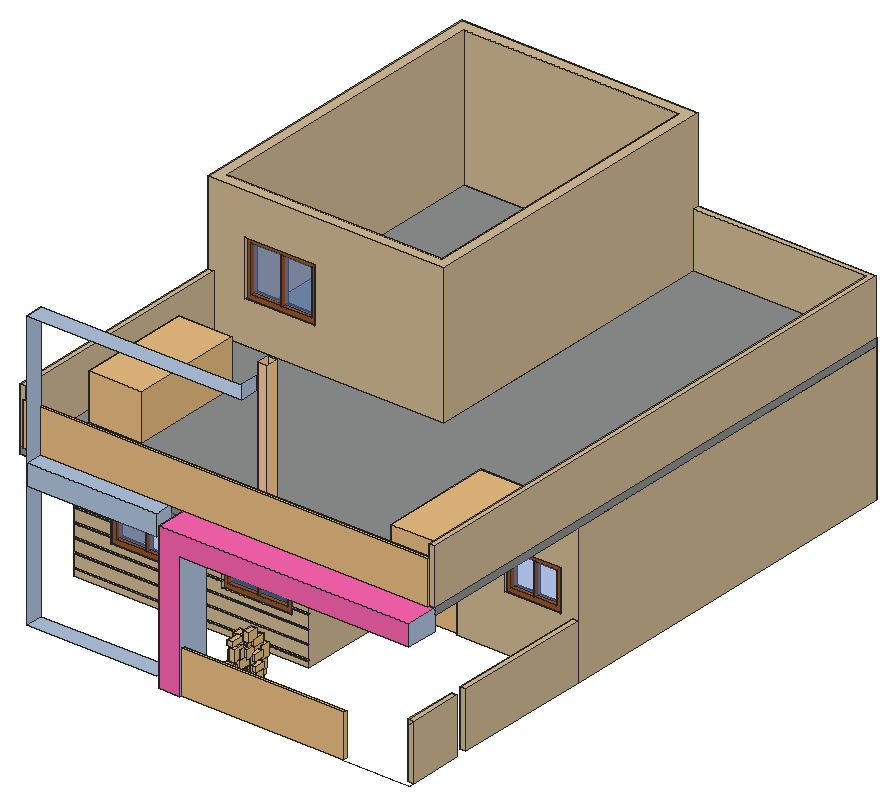
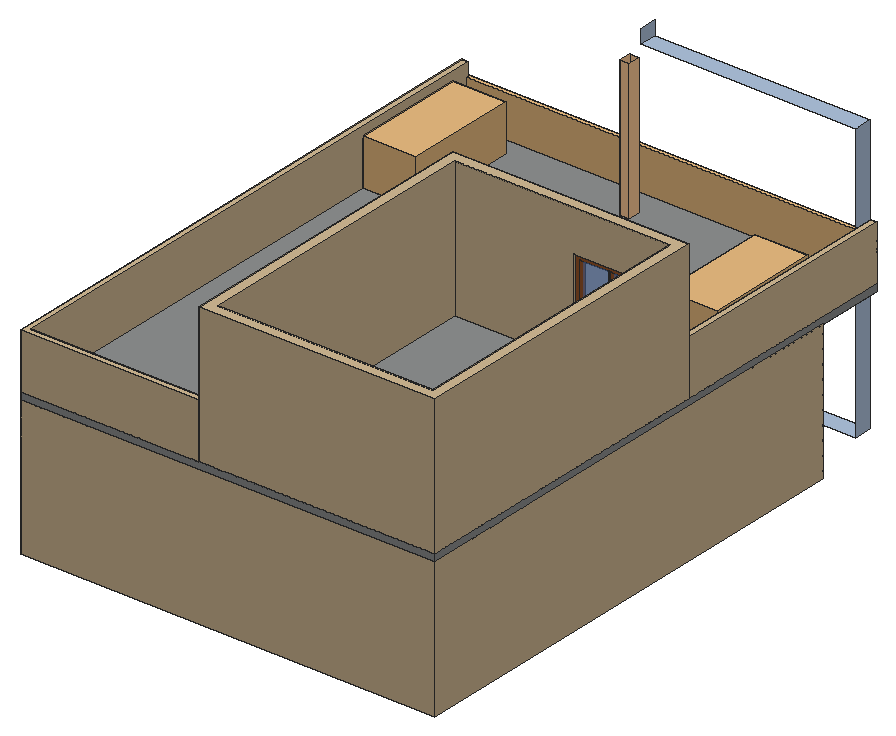
# SketchUp Ruby script. Lengths in inches.
U = 1.inch
M = Sketchup.active_model
def pt(a) = Geom::Point3d.new(a.map { |v| v * U })
def face(e, loops, mat)
  f = e.add_face(loops[0].map { |a| pt(a) })
  loops[1..].each { |l| e.add_face(l.map { |a| pt(a) }).erase! }
  f.material = f.back_material = mat if mat
  f
end
# faces: each face lists its corners as indices into pts; further lists are holes
def faces(e, pts, list, mat = nil) = list.each { |f| face(e, (f[0].is_a?(Array) ? f : [f]).map { |l| l.map { |i| pts[i] } }, mat) }
# xy, xz, yz: faces in a plane at the given z, y or x. An outline is a flat list of corners, or four numbers for a rectangle; further outlines are holes
def ring(l) = l.size == 4 ? [[l[0], l[1]], [l[2], l[1]], [l[2], l[3]], [l[0], l[3]]] : l.each_slice(2).to_a
def flat(e, list, mat, &to3) = list.each { |f| face(e, (f[0].is_a?(Array) ? f : [f]).map { |l| ring(l).map { |u, v| to3.(u, v) } }, mat) }
def xy(e, z, list, mat = nil) = flat(e, list, mat) { |x, y| [x, y, z] }
def xz(e, y, list, mat = nil) = flat(e, list, mat) { |x, z| [x, y, z] }
def yz(e, x, list, mat = nil) = flat(e, list, mat) { |y, z| [x, y, z] }
def lines(e, pts, list) = list.each { |a, b| e.add_line(pt(pts[a]), pt(pts[b])) }
# prism: a flat outline (further loops are holes) pulled along v
def prism(e, loops, v, mat = nil)
  f = face(e, loops, mat); d = Geom::Vector3d.new(v.map { |x| x * U })
  f.pushpull(f.normal.samedirection?(d) ? d.length : -d.length)
end
def box(e, o, s, mat = nil) = prism(e, [[o, [o[0] + s[0], o[1], o[2]], [o[0] + s[0], o[1] + s[1], o[2]], [o[0], o[1] + s[1], o[2]]]], [0, 0, s[2]], mat)
def at(x, y, z, deg = 0) = Geom::Transformation.translation(pt([x, y, z])) * Geom::Transformation.rotation(ORIGIN, Z_AXIS, deg.degrees)
def axes(o, x, y, z) = Geom::Transformation.new([*x, 0, *y, 0, *z, 0, *pt(o).to_a, 1])
def part(name) = M.definitions.add(name)
# library, detail: a bought-in or finely detailed component or shape, given as its bounding box
def library(name, o, s) = part(name).tap { |d| box(d.entities, o, s) }
def detail(e, o, s) = box(e.add_group.entities, o, s)
def put(e, d, t, mat = nil) = e.add_instance(d, t).tap { |i| i.material = mat if mat }
def group(e, t, mat = nil) = e.add_group.tap { |g| g.transformation = t; g.material = mat if mat }.entities
root = M.entities
M.materials.add("[0099_LightSteelBlue]").color = [176, 196, 222]
M.materials.add("[Blacktop Old 02]").color = [143, 145, 145]
M.materials.add("[Color A03]").color = [255, 101, 101]
M.materials.add("[Color C02]").color = [255, 204, 153]
M.materials.add("[Color K04]").color = [255, 50, 255]
M.materials.add("[Color L03]").color = [255, 101, 178]
M.materials.add("[Color M09]").color = [0, 0, 0]
M.materials.add("[Formica Beige]").color = [211, 187, 149]
M.materials.add("[Translucent Glass Blue]").color = [100, 149, 237]
M.materials["[Translucent Glass Blue]"].alpha = 0.5
M.materials.add("[Wood Cherry Original]").color = [152, 86, 42]
c1 = library("Untitled",[0,0,0],[36,4.39,84])
c2 = library("Group59\#1",[-32.98,33.92,22.15],[23.96,96.56,83.1])
c3 = library("Group60\#1",[-47.26,-81.53,115.8],[11.57,60.71,53.88])
c4 = library("Group61\#1",[17.15,84.19,16.4],[76.98,72.79,100.38])
c5 = library("Group62\#1",[-41.8,-20.16,82.85],[99.48,139.14,54.12])
c6 = library("Group63\#1",[-78.07,100.88,62.43],[61.26,81.43,86.37])
c7 = library("Group64\#1",[46.33,-12.9,51.95],[92.42,78.95,51.57])
c8 = library("Group65\#1",[-73.78,-20.03,120.09],[33.05,103.71,51.96])
c9 = library("Group66\#1",[-93.39,-19.9375,115.15],[70.74,15.37,89.07])
c10 = library("Group67\#1",[-160.6,-41.84,176.32],[92.55,73.84,45.89])
c11 = library("Group68\#1",[-72.58,-136.32,72.38],[80.41,85.97,95.72])
c12 = library("Group69\#1",[-107.89,47.83,91.71],[66.48,87.86,82.46])
c13 = library("Group70\#1",[-20.98,-42.53,-198.63],[46.69,46.24,172.61])
c14 = library("Group71\#1",[-0.8,-43.35,191.05],[81.04,80.57,74.82])
c15 = library("Group72\#1",[-44.16,-20.64,117.23],[64.94,35.73,104.26])
c16 = library("Group73\#2",[-85.2,-151.09,191.26],[83.6,108.34,38.47])
c17 = library("Group74\#1",[-43.32,-82.39,113.66],[8.74,67.58,95.91])
c18 = library("Group75\#1",[-19.52,-83.01,-122.96],[25.03,96.75,107.02])
c19 = library("Group76\#1",[-73.41,104.74,-36.57],[91.05,64.11,87.76])
c20 = library("Group77\#1",[6.72,-35.5625,-44.3],[97.86,50.43,71.28])
c21 = library("Group78\#1",[-46.16,95.67,-127.18],[89.22,60,98.58])
c22 = library("Group79\#1",[-73.36,-53.98,-265.87],[113.5,113.5,80.32])
c23 = library("Group80\#1",[-49.58,-31.64,-192.73],[34.2,35.75,335.89])
c24 = library("Group81\#1",[-33.25,31.15,20.5625],[19.21,100.94,38.88])
c25 = library("Group82\#1",[70.71,-26.24,-13.72],[94.01,86.31,40.81])
c26 = library("Group83\#1",[-78.76,-45.9375,-42.49],[89.36,13.07,73.45])
c27 = library("Group84\#1",[1.95,9.69,-124.66],[99.34,14.87,96.07])
c28 = library("Group85\#1",[5.34,-106.29,-47.41],[68.63,73.37,61.51])
c29 = library("Group86\#1",[4.23,10.03,-136.62],[40.98,41.87,51.36])
c30 = library("Group87\#1",[7.14,-44.59,-77.7],[48.84,15.98,59.8])
c31 = library("Group88\#1",[-32.7,-24.31,24.45],[55.13,61.32,79.5])
c32 = library("Group89\#1",[-77.24,-123.58,-46.56],[87.79,92.59,104.1])
c33 = library("Group90\#1",[-164.72,37.75,-20.84],[98.29,65.97,82.77])
c34 = library("Group91\#1",[-103.43,33.69,20.61],[71.41,32.36,40.62])
c35 = library("Group92\#1",[-125.68,-182.3125,23.5],[85.66,94.28,35.8])
c36 = library("Group93\#1",[5.2,-33.94,-67.23],[20.18,157.98,40.35])
c37 = library("Group94\#1",[2.39,9.02,-121.59],[42.15,71.34,93.56])
c38 = library("Group95\#1",[-55.3125,-129.29,-96.66],[79.37,72.9,68.93])
c39 = library("Group96\#1",[-140.7,-35.21,-77.44],[97.31,70.81,56.29])
c40 = library("Group97\#1",[-10.06,-56.42,72.68],[90.9,68.8,76.87])
c41 = library("Group98\#1",[12.8,58.29,-66.98],[80.58,78.21,79.14])
c42 = library("Group99\#1",[-35.4,-17.16,23.02],[118.23,50.83,58.94])
c43 = library("Group100\#1",[29.51,-171.04,-20.53],[91.11,101.22,39.04])
c44 = library("Group101\#1",[-97.95,11.13,-121.05],[102.09,51.91,53.69])
c45 = library("Group102\#1",[6.02,5.95,144.49],[89.45,87.47,55.68])
c46 = library("Group103\#1",[-45.73,-21.24,120.09],[87.14,68.72,79.33])
c47 = library("Group104\#1",[-32.38,-52.6,16.55],[60.96,98.07,53.51])
c48 = library("Group105\#1",[-69.28,-88.77,-223.3],[101.83,125.23,376.24])
c49 = library("Group106\#1",[-122.02,-42.04,23.03],[89.8,79.69,89.2])
c50 = library("Group107\#1",[-147.28,-98.05,24.68],[53.49,99.81,98.14])
c51 = library("Group108\#1",[38.95,-94,-129.36],[60.91,93.27,90.52])
c52 = library("Group109\#1",[-124.75,-75.19,-35.84],[77.11,72.51,79.94])
c53 = library("Group110\#1",[-78.58,0.56,-119.09],[84.31,12.02,77.58])
c54 = library("Group111\#1",[62.69,-31.6,-103.24],[86.45,84.15,71.79])
c55 = library("Group112\#1",[5.13,22.77,-174.65],[91.17,82.67,75.7])
c56 = library("Group113\#1",[-8.89,-115.37,23.85],[66.54,93.07,62.51])
c57 = library("Group114\#1",[-138.5625,33.88,-184.78],[81.4,51.14,109.21])
c58 = library("Group115\#1",[-39.22,1.8,-197.74],[25.16,42.04,242.32])
c59 = library("Group116\#1",[-16.77,0.31,-197.58],[31.04,19.97,97.43])
c60 = part("Group58\#1")
put(c60.entities,c2,at(0,0,0))
put(c60.entities,c3,at(0,0,0))
put(c60.entities,c4,at(0,0,0))
put(c60.entities,c5,at(0,0,0))
put(c60.entities,c6,at(0,0,0))
put(c60.entities,c7,at(0,0,0))
put(c60.entities,c8,at(0,0,0))
put(c60.entities,c9,at(0,0,0))
put(c60.entities,c10,at(0,0,0))
put(c60.entities,c11,at(0,0,0))
put(c60.entities,c12,at(0,0,0))
put(c60.entities,c13,at(0,0,0))
put(c60.entities,c14,at(0,0,0))
put(c60.entities,c15,at(0,0,0))
put(c60.entities,c16,at(0,0,0))
put(c60.entities,c17,at(0,0,0))
put(c60.entities,c18,at(0,0,0))
put(c60.entities,c19,at(0,0,0))
put(c60.entities,c20,at(0,0,0))
put(c60.entities,c21,at(0,0,0))
put(c60.entities,c22,at(0,0,0))
put(c60.entities,c23,at(0,0,0))
put(c60.entities,c24,at(0,0,0))
put(c60.entities,c25,at(0,0,0))
put(c60.entities,c26,at(0,0,0))
put(c60.entities,c27,at(0,0,0))
put(c60.entities,c28,at(0,0,0))
put(c60.entities,c29,at(0,0,0))
put(c60.entities,c30,at(0,0,0))
put(c60.entities,c31,at(0,0,0))
put(c60.entities,c32,at(0,0,0))
put(c60.entities,c33,at(0,0,0))
put(c60.entities,c34,at(0,0,0))
put(c60.entities,c35,at(0,0,0))
put(c60.entities,c36,at(0,0,0))
put(c60.entities,c37,at(0,0,0))
put(c60.entities,c38,at(0,0,0))
put(c60.entities,c39,at(0,0,0))
put(c60.entities,c40,at(0,0,0))
put(c60.entities,c41,at(0,0,0))
put(c60.entities,c42,at(0,0,0))
put(c60.entities,c43,at(0,0,0))
put(c60.entities,c44,at(0,0,0))
put(c60.entities,c45,at(0,0,0))
put(c60.entities,c46,at(0,0,0))
put(c60.entities,c47,at(0,0,0))
put(c60.entities,c48,at(0,0,0))
put(c60.entities,c49,at(0,0,0))
put(c60.entities,c50,at(0,0,0))
put(c60.entities,c51,at(0,0,0))
put(c60.entities,c52,at(0,0,0))
put(c60.entities,c53,at(0,0,0))
put(c60.entities,c54,at(0,0,0))
put(c60.entities,c55,at(0,0,0))
put(c60.entities,c56,at(0,0,0))
put(c60.entities,c57,at(0,0,0))
put(c60.entities,c58,at(0,0,0))
put(c60.entities,c59,at(0,0,0))
c61 = part("SimLab\#1")
put(c61.entities,c60,at(0,0,0))
c62 = part("Group23\#2")
xy(c62.entities,0,[[-20.0625,-14.0625,-0.59,14.0625],[0.59,-14.0625,20.0625,14.0625]])
c63 = part("Group22\#1")
prism(c63.entities,[[[-24,-18,0],[-24,18,0],[24,18,0],[24,-18,0]],[[-0.59,14.0625,0],[-20.0625,14.0625,0],[-20.0625,-14.0625,0],[-0.59,-14.0625,0]],[[0.59,-14.0625,0],[20.0625,-14.0625,0],[20.0625,14.0625,0],[0.59,14.0625,0]]],[0,0,5.875])
put(c63.entities,c62,at(0,0,2.9375),"[Translucent Glass Blue]")
c64 = part("Group39\#1")
prism(c64.entities,[[[1377.99,-24.125,126.61],[1377.99,-24.125,174.61],[1377.99,98,174],[1377.99,98,126]]],[5,0,0])
c65 = part("Group40\#1")
box(c65.entities,[1377.99,-79.96,126],[5,46.83,48])
c66 = library("Group\#12",[0,0,0],[143.15,3.15,36.98])
c67 = part("Group25\#2")
xy(c67.entities,0,[[-26.0625,-20.0625,-0.59,20.0625],[0.59,-20.0625,26.0625,20.0625]])
c68 = part("Group24\#1")
prism(c68.entities,[[[-30,24,0],[30,24,0],[30,-24,0],[-30,-24,0]],[[26.0625,20.0625,0],[0.59,20.0625,0],[0.59,-20.0625,0],[26.0625,-20.0625,0]],[[-0.59,-20.0625,0],[-0.59,20.0625,0],[-26.0625,20.0625,0],[-26.0625,-20.0625,0]]],[0,0,5.875])
put(c68.entities,c67,at(0,0,2.9375),"[Translucent Glass Blue]")
c69 = part("Group27\#2")
xy(c69.entities,0,[[-26.0625,-20.0625,-0.59,20.0625],[0.59,-20.0625,26.0625,20.0625]])
c70 = part("Group26\#1")
prism(c70.entities,[[[30,-24,0],[-30,-24,0],[-30,24,0],[30,24,0]],[[0.59,20.0625,0],[0.59,-20.0625,0],[26.0625,-20.0625,0],[26.0625,20.0625,0]],[[-0.59,20.0625,0],[-26.0625,20.0625,0],[-26.0625,-20.0625,0],[-0.59,-20.0625,0]]],[0,0,5.875])
put(c70.entities,c69,at(0,0,2.9375),"[Translucent Glass Blue]")
c71 = library("SKT_Nearly Natural 5' Kentia Palm Silk Tree",[-23.18,-17.61,0],[47.48,43.95,59.125])
c72 = part("Group31\#2")
xy(c72.entities,0,[[-26.0625,-20.0625,-0.59,20.0625],[0.59,-20.0625,26.0625,20.0625]])
c73 = part("Group30\#1")
prism(c73.entities,[[[-30,24,0],[30,24,0],[30,-24,0],[-30,-24,0]],[[-0.59,20.0625,0],[-26.0625,20.0625,0],[-26.0625,-20.0625,0],[-0.59,-20.0625,0]],[[0.59,20.0625,0],[0.59,-20.0625,0],[26.0625,-20.0625,0],[26.0625,20.0625,0]]],[0,0,5.875])
put(c73.entities,c72,at(0,0,2.9375),"[Translucent Glass Blue]")
c74 = part("Group43\#1")
prism(c74.entities,[[[1377.99,-57.52,252],[1377.99,415,252],[1228.34,415,252],[1228.34,420,252],[1382.99,420,252],[1382.99,-57.52,252]]],[0,0,48])
c75 = part("Group44\#1")
box(c75.entities,[1024.5625,-57.52,252],[5,203.11,48])
c76 = library("Group\#13",[0,0,0],[357.37,3.15,36.98])
xy(root,126,[[142.05,102.625,160.13,130.0625]])
xy(root,126,[[18,114.625,130.05,130.0625]],"[0099_LightSteelBlue]")
xy(root,234,[[160.13,102.625,358.43,130.0625]],"[0099_LightSteelBlue]")
xy(root,246,[[24.2,362.83,25.75,363.08,27.17,363.73,28.38,364.73,29.29,366,29.84,367.47,30,369.02,29.74,370.57,29.09,372,28.1,373.21,26.82,374.12,25.36,374.67,23.8,374.82,22.25,374.5625,20.83,373.91,19.62,372.92,18.71,371.65,18.16,370.18,18,368.62,18.26,367.08,18.91,365.65,19.9,364.4375,21.18,363.53,22.64,362.98],[86.29,362.83,87.83,363.08,89.26,363.73,90.47,364.73,91.38,366,91.93,367.47,92.08,369.02,91.83,370.57,91.18,372,90.18,373.21,88.91,374.12,87.44,374.67,85.88,374.82,84.34,374.5625,82.91,373.91,81.7,372.92,80.79,371.65,80.24,370.18,80.09,368.62,80.35,367.08,80.99,365.65,81.99,364.4375,83.26,363.53,84.73,362.98],[148.375,362.83,149.92,363.08,151.35,363.73,152.55,364.73,153.47,366,154.02,367.47,154.17,369.02,153.91,370.57,153.26,372,152.27,373.21,150.99,374.12,149.53,374.67,147.97,374.82,146.42,374.5625,145,373.91,143.79,372.92,142.88,371.65,142.33,370.18,142.18,368.62,142.43,367.08,143.08,365.65,144.07,364.4375,145.35,363.53,146.82,362.98],[210.46,362.83,212,363.08,213.43,363.73,214.64,364.73,215.55,366,216.1,367.47,216.25,369.02,216,370.57,215.35,372,214.35,373.21,213.08,374.12,211.61,374.67,210.06,374.82,208.51,374.5625,207.08,373.91,205.875,372.92,204.96,371.65,204.41,370.18,204.26,368.62,204.52,367.08,205.17,365.65,206.16,364.4375,207.43,363.53,208.9,362.98],[272.55,362.83,274.09,363.08,275.52,363.73,276.73,364.73,277.64,366,278.1875,367.47,278.34,369.02,278.08,370.57,277.44,372,276.44,373.21,275.17,374.12,273.7,374.67,272.14,374.82,270.6,374.5625,269.17,373.91,267.96,372.92,267.05,371.65,266.5,370.18,266.35,368.62,266.6,367.08,267.25,365.65,268.25,364.4375,269.52,363.53,270.99,362.98],
  [334.63,362.83,336.18,363.08,337.6,363.73,338.8125,364.73,339.72,366,340.27,367.47,340.43,369.02,340.17,370.57,339.52,372,338.53,373.21,337.25,374.12,335.79,374.67,334.23,374.82,332.68,374.5625,331.26,373.91,330.05,372.92,329.13,371.65,328.58,370.18,328.43,368.62,328.6875,367.08,329.34,365.65,330.33,364.4375,331.61,363.53,333.07,362.98],[24.2,577.59,25.75,577.84,27.17,578.49,28.38,579.49,29.29,580.76,29.84,582.23,30,583.78,29.74,585.33,29.09,586.76,28.1,587.97,26.82,588.875,25.36,589.43,23.8,589.58,22.25,589.32,20.83,588.67,19.62,587.68,18.71,586.41,18.16,584.9375,18,583.38,18.26,581.83,18.91,580.41,19.9,579.2,21.18,578.29,22.64,577.74],[86.29,577.59,87.83,577.84,89.26,578.49,90.47,579.49,91.38,580.76,91.93,582.23,92.08,583.78,91.83,585.33,91.18,586.76,90.18,587.97,88.91,588.875,87.44,589.43,85.88,589.58,84.34,589.32,82.91,588.67,81.7,587.68,80.79,586.41,80.24,584.9375,80.09,583.38,80.35,581.83,80.99,580.41,81.99,579.2,83.26,578.29,84.73,577.74],[148.375,577.59,149.92,577.84,151.35,578.49,152.55,579.49,153.47,580.76,154.02,582.23,154.17,583.78,153.91,585.33,153.26,586.76,152.27,587.97,150.99,588.875,149.53,589.43,147.97,589.58,146.42,589.32,145,588.67,143.79,587.68,142.88,586.41,142.33,584.9375,142.18,583.38,142.43,581.83,143.08,580.41,144.07,579.2,145.35,578.29,146.82,577.74],[210.46,577.59,212,577.84,213.43,578.49,214.64,579.49,215.55,580.76,216.1,582.23,216.25,583.78,216,585.33,215.35,586.76,214.35,587.97,213.08,588.875,211.61,589.43,210.06,589.58,208.51,589.32,207.08,588.67,205.875,587.68,204.96,586.41,204.41,584.9375,204.26,583.38,204.52,581.83,205.17,580.41,206.16,579.2,207.43,578.29,208.9,577.74],
  [272.55,577.59,274.09,577.84,275.52,578.49,276.73,579.49,277.64,580.76,278.1875,582.23,278.34,583.78,278.08,585.33,277.44,586.76,276.44,587.97,275.17,588.875,273.7,589.43,272.14,589.58,270.6,589.32,269.17,588.67,267.96,587.68,267.05,586.41,266.5,584.9375,266.35,583.38,266.6,581.83,267.25,580.41,268.25,579.2,269.52,578.29,270.99,577.74],[334.63,577.59,336.18,577.84,337.6,578.49,338.8125,579.49,339.72,580.76,340.27,582.23,340.43,583.78,340.17,585.33,339.52,586.76,338.53,587.97,337.25,588.875,335.79,589.43,334.23,589.58,332.68,589.32,331.26,588.67,330.05,587.68,329.13,586.41,328.58,584.9375,328.43,583.38,328.6875,581.83,329.34,580.41,330.33,579.2,331.61,578.29,333.07,577.74]])
xy(root,252,[[186.48,154.03,194.3,164.47]],"[0099_LightSteelBlue]")
xy(root,252,[[142.05,102.625,358.43,130.0625]],"[Color L03]")
xy(root,366,[[18,114.625,203.78,130.0625]],"[0099_LightSteelBlue]")
xz(root,102.625,[[142.05,126,160.13,126,160.13,234,358.43,234,358.43,252,142.05,252]],"[Color L03]")
xz(root,130.0625,[[142.05,126,142.05,252,358.43,252,358.43,234,160.13,234,160.13,126]])
xz(root,154.03,[[186.48,252,194.3,372]],"[Color C02]")
xz(root,164.47,[[186.48,252,194.3,372]],"[Color C02]")
yz(root,18,[[114.625,126,130.0625,366]],"[0099_LightSteelBlue]")
yz(root,142.05,[[102.625,126,130.0625,252]],"[Color L03]")
yz(root,160.13,[[102.625,126,130.0625,234]],"[0099_LightSteelBlue]")
yz(root,186.48,[[154.03,252,164.47,372]],"[Color C02]")
yz(root,194.3,[[154.03,252,164.47,372]],"[Color C02]")
yz(root,203.78,[[114.625,366,130.0625,378]],"[0099_LightSteelBlue]")
yz(root,358.43,[[102.625,234,130.0625,252]],"[0099_LightSteelBlue]")
p = [[31.9375,192.08,162],[31.9375,192.08,210],[91.9375,192.08,210],[91.9375,192.08,162],[128.47,192.08,162],[128.47,192.08,210],
  [188.47,192.08,210],[188.47,192.08,162],[358.43,102.625,126],[358.43,107.625,126],[299.35,107.625,126],[299.35,102.625,126],
  [358.43,102.625,174],[358.43,107.625,174]]
lines(root,p,[[0,1],[1,2],[2,3],[3,0],[4,5],[5,6],[6,7],[7,4],[8,9],[10,11],[11,8],[12,13]])
put(root,c1,at(217.22,287.67,126))
put(root,c61,axes([199.88,125.74,154.35],[0.05714,0,0],[0,0.10569,0],[0,0,0.10662]))
g1 = group(root,at(0,187.58,126),"[Formica Beige]")
xy(g1,0,[[0,0,0,420,358.43,420,358.43,98,253.22,98,253.22,107,349.43,107,349.43,411,9,411,9,9,194.78,9,194.78,107,217.22,107,217.22,98,203.78,98,203.78,0]])
xy(g1,5.17,[[0,0,203.78,1]])
xy(g1,7.11,[[0,0,203.78,1]])
xy(g1,16.99,[[0,0,203.78,1]])
xy(g1,18.92,[[0,0,203.78,1]])
xy(g1,28.8,[[0,0,203.78,1]])
xy(g1,30.74,[[0,0,203.78,1]])
xy(g1,36,[[31.9375,0,91.9375,9],[128.47,0,188.47,9]])
xy(g1,40.61,[[0,0,31.9375,1],[91.9375,0,128.47,1],[188.47,0,203.78,1]])
xy(g1,42.55,[[0,0,31.9375,1],[91.9375,0,128.47,1],[188.47,0,203.78,1]])
xy(g1,48,[[294.74,98,342.74,102.5],[294.74,102.5,342.74,107]])
xy(g1,52.42,[[0,0,31.9375,1],[91.9375,0,128.47,1],[188.47,0,203.78,1]])
xy(g1,54.36,[[0,0,31.9375,1],[91.9375,0,128.47,1],[188.47,0,203.78,1]])
xy(g1,64.24,[[0,0,31.9375,1],[91.9375,0,128.47,1],[188.47,0,203.78,1]])
xy(g1,66.17,[[0,0,31.9375,1],[91.9375,0,128.47,1],[188.47,0,203.78,1]])
xy(g1,76.05,[[0,0,31.9375,1],[91.9375,0,128.47,1],[188.47,0,203.78,1]])
xy(g1,77.99,[[0,0,31.9375,1],[91.9375,0,128.47,1],[188.47,0,203.78,1]])
xy(g1,84,[[31.9375,0,91.9375,9],[128.47,0,188.47,9],[217.22,98,253.22,107],[294.74,98,342.74,102.5],[294.74,102.5,342.74,107]])
xy(g1,87.86,[[0,0,203.78,1]])
xy(g1,89.8,[[0,0,203.78,1]])
xy(g1,99.67,[[0,0,203.78,1]])
xy(g1,101.61,[[0,0,203.78,1]])
xy(g1,111.49,[[0,0,203.78,1]])
xy(g1,113.42,[[0,0,203.78,1]])
xy(g1,120,[[[0,0,203.78,0,203.78,98,358.43,98,358.43,420,0,420],[9,9,9,411,349.43,411,349.43,107,194.78,107,194.78,9]]])
xz(g1,0,[[0,0,203.78,5.17],[0,7.11,203.78,16.99],[0,18.92,203.78,28.8],[0,30.74,203.78,30.74,203.78,40.61,188.47,40.61,188.47,36,128.47,36,128.47,40.61,91.9375,40.61,91.9375,36,31.9375,36,31.9375,40.61,0,40.61],[0,42.55,31.9375,52.42],
  [91.9375,42.55,128.47,52.42],[188.47,42.55,203.78,52.42],[0,54.36,31.9375,64.24],[91.9375,54.36,128.47,64.24],[188.47,54.36,203.78,64.24],
  [0,66.17,31.9375,76.05],[91.9375,66.17,128.47,76.05],[188.47,66.17,203.78,76.05],[0,77.99,31.9375,77.99,31.9375,84,91.9375,84,91.9375,77.99,128.47,77.99,128.47,84,188.47,84,188.47,77.99,203.78,77.99,203.78,87.86,0,87.86],[0,89.8,203.78,99.67],
  [0,101.61,203.78,111.49],[0,113.42,203.78,120]])
xz(g1,1,[[0,5.17,203.78,7.11],[0,16.99,203.78,18.92],[0,28.8,203.78,30.74],[0,40.61,31.9375,42.55],[91.9375,40.61,128.47,42.55],
  [188.47,40.61,203.78,42.55],[0,52.42,31.9375,54.36],[91.9375,52.42,128.47,54.36],[188.47,52.42,203.78,54.36],[0,64.24,31.9375,66.17],
  [91.9375,64.24,128.47,66.17],[188.47,64.24,203.78,66.17],[0,76.05,31.9375,77.99],[91.9375,76.05,128.47,77.99],[188.47,76.05,203.78,77.99],
  [0,87.86,203.78,89.8],[0,99.67,203.78,101.61],[0,111.49,203.78,113.42]])
xz(g1,9,[[[9,0,194.78,120],[31.9375,36,91.9375,84],[128.47,36,188.47,84]]])
xz(g1,98,[[[203.78,0,217.22,0,217.22,84,253.22,84,253.22,0,358.43,0,358.43,120,203.78,120],[294.74,48,342.74,84]]])
xz(g1,107,[[[194.78,0,194.78,120,349.43,120,349.43,0,253.22,0,253.22,84,217.22,84,217.22,0],[294.74,48,342.74,84]]])
xz(g1,411,[[9,0,349.43,120]])
xz(g1,420,[[0,0,358.43,120]])
yz(g1,0,[[0,0,0,5.17,1,5.17,1,7.11,0,7.11,0,16.99,1,16.99,1,18.92,0,18.92,0,28.8,1,28.8,1,30.74,0,30.74,0,40.61,1,40.61,1,42.55,0,42.55,0,52.42,1,52.42,1,54.36,0,54.36,0,64.24,1,64.24,1,66.17,0,66.17,0,76.05,1,76.05,1,77.99,0,77.99,0,87.86,1,87.86,1,89.8,0,89.8,0,99.67,1,99.67,1,101.61,0,101.61,0,111.49,1,111.49,1,113.42,0,113.42,0,120,420,120,420,0],[0,5.17,1,7.11],[0,16.99,1,18.92],[0,28.8,1,30.74],[0,40.61,1,42.55],
  [0,52.42,1,54.36],[0,64.24,1,66.17],[0,76.05,1,77.99],[0,87.86,1,89.8],[0,99.67,1,101.61],
  [0,111.49,1,113.42]])
yz(g1,9,[[9,0,411,120]])
yz(g1,31.9375,[[0,36,9,36,9,84,0,84,0,77.99,1,77.99,1,76.05,0,76.05,0,66.17,1,66.17,1,64.24,0,64.24,0,54.36,1,54.36,1,52.42,0,52.42,0,42.55,1,42.55,1,40.61,0,40.61],[0,40.61,1,42.55],[0,52.42,1,54.36],[0,64.24,1,66.17],[0,76.05,1,77.99]])
yz(g1,91.9375,[[0,36,0,40.61,1,40.61,1,42.55,0,42.55,0,52.42,1,52.42,1,54.36,0,54.36,0,64.24,1,64.24,1,66.17,0,66.17,0,76.05,1,76.05,1,77.99,0,77.99,0,84,9,84,9,36],[0,40.61,1,42.55],[0,52.42,1,54.36],[0,64.24,1,66.17],[0,76.05,1,77.99]])
yz(g1,128.47,[[0,36,9,36,9,84,0,84,0,77.99,1,77.99,1,76.05,0,76.05,0,66.17,1,66.17,1,64.24,0,64.24,0,54.36,1,54.36,1,52.42,0,52.42,0,42.55,1,42.55,1,40.61,0,40.61],[0,40.61,1,42.55],[0,52.42,1,54.36],[0,64.24,1,66.17],[0,76.05,1,77.99]])
yz(g1,188.47,[[0,36,0,40.61,1,40.61,1,42.55,0,42.55,0,52.42,1,52.42,1,54.36,0,54.36,0,64.24,1,64.24,1,66.17,0,66.17,0,76.05,1,76.05,1,77.99,0,77.99,0,84,9,84,9,36],[0,40.61,1,42.55],[0,52.42,1,54.36],[0,64.24,1,66.17],[0,76.05,1,77.99]])
yz(g1,194.78,[[9,0,107,120]])
yz(g1,203.78,[[0,0,98,0,98,120,0,120,0,113.42,1,113.42,1,111.49,0,111.49,0,101.61,1,101.61,1,99.67,0,99.67,0,89.8,1,89.8,1,87.86,0,87.86,0,77.99,1,77.99,1,76.05,0,76.05,0,66.17,1,66.17,1,64.24,0,64.24,0,54.36,1,54.36,1,52.42,0,52.42,0,42.55,1,42.55,1,40.61,0,40.61,0,30.74,1,30.74,1,28.8,0,28.8,0,18.92,1,18.92,1,16.99,0,16.99,0,7.11,1,7.11,1,5.17,0,5.17],[0,5.17,1,7.11],[0,16.99,1,18.92],[0,28.8,1,30.74],[0,40.61,1,42.55],
  [0,52.42,1,54.36],[0,64.24,1,66.17],[0,76.05,1,77.99],[0,87.86,1,89.8],[0,99.67,1,101.61],
  [0,111.49,1,113.42]])
yz(g1,217.22,[[98,0,107,84]])
yz(g1,253.22,[[98,0,107,84]])
yz(g1,294.74,[[98,48,102.5,84],[102.5,48,107,84]])
yz(g1,342.74,[[98,48,102.5,84],[102.5,48,107,84]])
yz(g1,349.43,[[107,0,411,120]])
yz(g1,358.43,[[98,0,420,120]])
put(g1,c63,axes([318.74,99.5625,66],[-1,0,0],[0,0,1],[0,1,0]),"[Wood Cherry Original]")
put(root,c64,at(-1024.5625,187.58,0),"[Formica Beige]")
put(root,c65,at(-1024.5625,187.58,0),"[Formica Beige]")
put(root,c66,at(158.16,103.55,126))
put(root,c68,axes([158.47,195.02,186],[1,0,0],[0,0,1],[0,-1,0]),"[Wood Cherry Original]")
put(root,c70,axes([61.9375,195.02,186],[1,0,0],[0,0,1],[0,-1,0]),"[Wood Cherry Original]")
g2 = group(root,at(18,114.625,234),"[0099_LightSteelBlue]")
box(g2,[0,0,0],[112.05,15.4375,18])
g3 = group(root,at(0,187.58,246),"[Color K04]")
xy(g3,0,[[0,-57.52,358.43,420]],"[Color A03]")
xy(g3,6,[[0,-57.52,358.43,420]],"[Blacktop Old 02]")
xz(g3,-57.52,[[0,0,358.43,6]],"[Blacktop Old 02]")
xz(g3,420,[[0,0,358.43,6]],"[Blacktop Old 02]")
yz(g3,0,[[-57.52,0,420,6]],"[Blacktop Old 02]")
yz(g3,358.43,[[-57.52,0,420,6]],"[Blacktop Old 02]")
put(root,c71,axes([329.85,185.13,252],[0.97,0,0],[0,2.2136,0],[0,0,0.67493]))
g4 = group(root,at(0,333.17,252),"[Formica Beige]")
xy(g4,0,[[0,0,0,274.41,9,274.41,9,9,194.78,9,194.78,107,203.78,107,203.78,0],[194.78,107,203.78,265.41],[9,265.41,203.78,274.41]])
xy(g4,36,[[31.9375,0,91.9375,4.5],[31.9375,4.5,91.9375,9]])
xy(g4,84,[[31.9375,0,91.9375,4.5],[31.9375,4.5,91.9375,9]])
xy(g4,120,[[[0,0,203.78,274.41],[9,9,194.78,265.41]]])
xz(g4,0,[[[0,0,203.78,120],[31.9375,36,91.9375,84]]])
xz(g4,9,[[[9,0,194.78,120],[31.9375,36,91.9375,84]]])
xz(g4,265.41,[[9,0,194.78,120]])
xz(g4,274.41,[[0,0,203.78,120]])
yz(g4,0,[[0,0,274.41,120]])
yz(g4,9,[[9,0,265.41,120]])
yz(g4,31.9375,[[0,36,4.5,84],[4.5,36,9,84]])
yz(g4,91.9375,[[0,36,4.5,84],[4.5,36,9,84]])
yz(g4,194.78,[[9,0,265.41,120]])
yz(g4,203.78,[[0,0,274.41,120]])
put(g4,c73,axes([61.9375,1.5625,60],[-1,0,0],[0,0,1],[0,1,0]),"[Wood Cherry Original]")
put(root,c74,at(-1024.5625,187.58,0),"[Formica Beige]")
put(root,c75,at(-1024.5625,187.58,0),"[Formica Beige]")
put(root,c76,axes([3.03,128.49,252],[0.9805,0,0],[0,1,0],[0,0,1]),"[Color M09]")
put(root,c71,axes([38.49,222.96,252.14],[0.97,0,0],[0,2.2136,0],[0,0,0.67493]))
